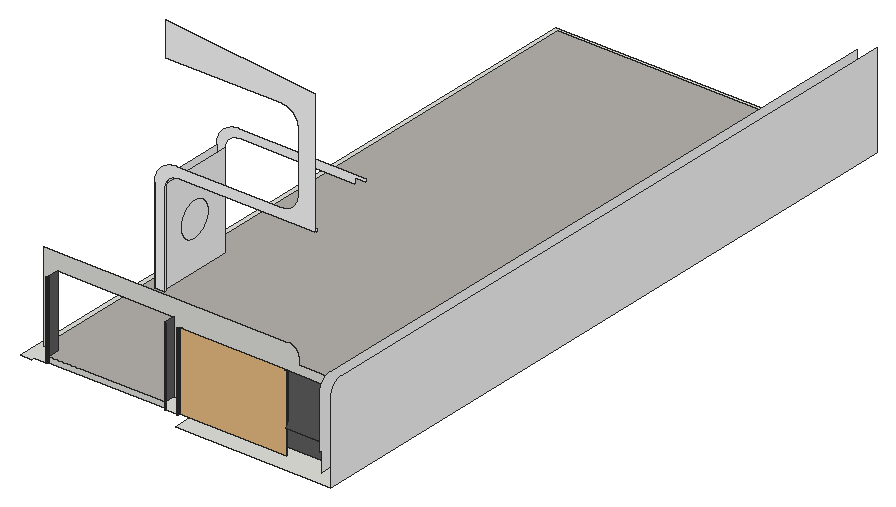
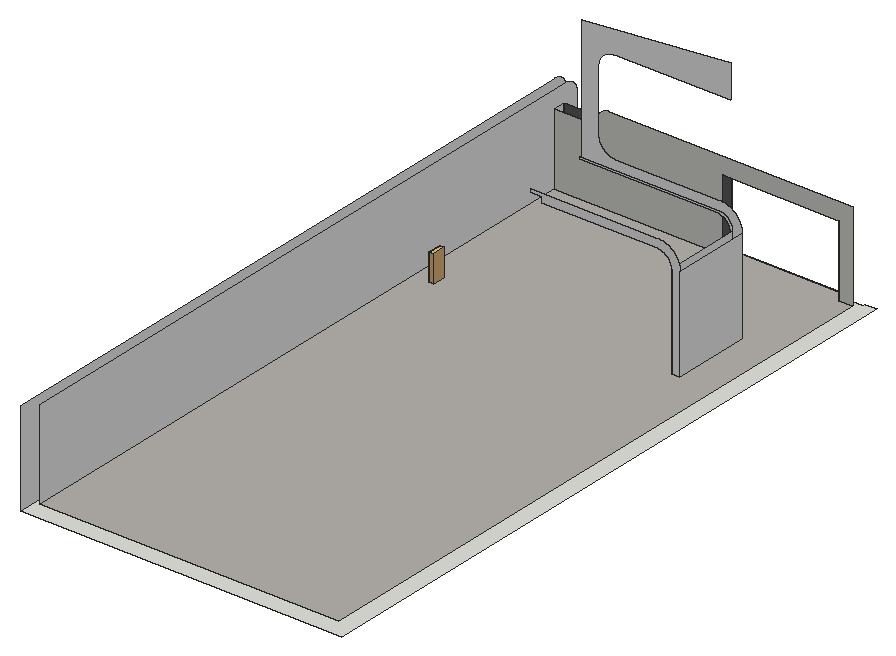
# SketchUp Ruby script. Lengths in inches.
U = 1.inch
M = Sketchup.active_model
def pt(a) = Geom::Point3d.new(a.map { |v| v * U })
def face(e, loops, mat)
  f = e.add_face(loops[0].map { |a| pt(a) })
  loops[1..].each { |l| e.add_face(l.map { |a| pt(a) }).erase! }
  f.material = f.back_material = mat if mat
  f
end
# faces: each face lists its corners as indices into pts; further lists are holes
def faces(e, pts, list, mat = nil) = list.each { |f| face(e, (f[0].is_a?(Array) ? f : [f]).map { |l| l.map { |i| pts[i] } }, mat) }
# xy, xz, yz: faces in a plane at the given z, y or x. An outline is a flat list of corners, or four numbers for a rectangle; further outlines are holes
def ring(l) = l.size == 4 ? [[l[0], l[1]], [l[2], l[1]], [l[2], l[3]], [l[0], l[3]]] : l.each_slice(2).to_a
def flat(e, list, mat, &to3) = list.each { |f| face(e, (f[0].is_a?(Array) ? f : [f]).map { |l| ring(l).map { |u, v| to3.(u, v) } }, mat) }
def xy(e, z, list, mat = nil) = flat(e, list, mat) { |x, y| [x, y, z] }
def xz(e, y, list, mat = nil) = flat(e, list, mat) { |x, z| [x, y, z] }
def yz(e, x, list, mat = nil) = flat(e, list, mat) { |y, z| [x, y, z] }
def lines(e, pts, list) = list.each { |a, b| e.add_line(pt(pts[a]), pt(pts[b])) }
# prism: a flat outline (further loops are holes) pulled along v
def prism(e, loops, v, mat = nil)
  f = face(e, loops, mat); d = Geom::Vector3d.new(v.map { |x| x * U })
  f.pushpull(f.normal.samedirection?(d) ? d.length : -d.length)
end
def box(e, o, s, mat = nil) = prism(e, [[o, [o[0] + s[0], o[1], o[2]], [o[0] + s[0], o[1] + s[1], o[2]], [o[0], o[1] + s[1], o[2]]]], [0, 0, s[2]], mat)
def at(x, y, z, deg = 0) = Geom::Transformation.translation(pt([x, y, z])) * Geom::Transformation.rotation(ORIGIN, Z_AXIS, deg.degrees)
def axes(o, x, y, z) = Geom::Transformation.new([*x, 0, *y, 0, *z, 0, *pt(o).to_a, 1])
def part(name) = M.definitions.add(name)
# library, detail: a bought-in or finely detailed component or shape, given as its bounding box
def library(name, o, s) = part(name).tap { |d| box(d.entities, o, s) }
def detail(e, o, s) = box(e.add_group.entities, o, s)
def put(e, d, t, mat = nil) = e.add_instance(d, t).tap { |i| i.material = mat if mat }
def group(e, t, mat = nil) = e.add_group.tap { |g| g.transformation = t; g.material = mat if mat }.entities
root = M.entities
M.materials.add("1421 AP 8232 ELEGANT GREY").color = [96, 96, 96]
M.materials.add("[Quartz Light Grey]").color = [251, 251, 252]
M.materials.add("[Tile Travertine 2 inch]").color = [181, 178, 172]
c1 = library("Group\#28",[0,-0.25,0],[115.92,0.25,83.97])
c2 = library("Group\#141",[-208.23,2037.18,75.37],[621.09,225.61,1251.82])
xy(root,-18,[[180,36,180,55,169,55,169,54.92,168.99,54.84,168.99,54.76,168.98,54.6875,168.96,54.61,168.94,54.53,168.92,54.46,168.9,54.38,168.875,54.31,168.85,54.23,168.82,54.16,168.74,54.02,168.71,53.96,168.66,53.89,168.62,53.82,168.47,53.64,168.41,53.59,168.36,53.53,168.18,53.38,168.11,53.34,168.04,53.29,167.98,53.26,167.84,53.18,167.77,53.15,167.69,53.125,167.62,53.1,167.54,53.08,167.47,53.06,167.39,53.04,167.3125,53.02,167.24,53.01,167.16,53.01,167.08,53,154.92,53,154.84,53.01,154.76,53.01,154.6875,53.02,154.61,53.04,154.53,53.06,154.46,53.08,154.38,53.1,154.31,53.125,154.23,53.15,154.16,53.18,154.02,53.26,153.96,53.29,153.89,53.34,153.82,53.38,153.64,53.53,153.59,53.59,153.53,53.64,153.38,53.82,153.34,53.89,153.29,53.96,153.26,54.02,153.18,54.16,153.15,54.23,153.125,54.31,153.1,54.38,153.08,54.46,153.06,54.53,153.04,54.61,153.02,54.6875,153.01,54.76,153.01,54.84,153,54.92,153,55,27,55,27,54.92,26.99,54.84,26.99,54.76,26.98,54.6875,26.96,54.61,26.94,54.53,26.92,54.46,26.9,54.38,26.875,54.31,26.85,54.23,26.82,54.16,26.74,54.02,26.71,53.96,26.66,53.89,26.62,53.82,26.47,53.64,26.41,53.59,26.36,53.53,26.18,53.38,26.11,53.34,26.04,53.29,25.98,53.26,25.84,53.18,25.77,53.15,25.69,53.125,25.62,53.1,25.54,53.08,25.47,53.06,25.39,53.04,25.3125,53.02,25.24,53.01,25.16,53.01,25.08,53,12,53,12,50,0,50,0,775,348,775,348,36]])
xy(root,-12,[[27,55,153,55,153,67,336,67,336,763,12,763,12,67,27,67]],"[Tile Travertine 2 inch]")
xy(root,0,[[36,187,36,271,45,271,45,189,47,189,47,187]],"[Quartz Light Grey]")
xy(root,9.97,[[284.92,53.5,336,55]])
xz(root,53,[[154.92,-18,155,66]],"1421 AP 8232 ELEGANT GREY")
xz(root,53.01,[[25.16,-18,25.24,66],[154.76,-18,154.84,66],[167.16,-18,167.24,65.97]],"1421 AP 8232 ELEGANT GREY")
xz(root,53.5,[[284.92,9.97,336,9.97,336,66,288,66,288,17.6875,287.99,17.53,287.98,17.37,287.97,17.22,287.95,16.9,287.93,16.75,287.92,16.59,287.9,16.43,287.875,16.28,287.85,16.12,287.83,15.97,287.8,15.8125,287.77,15.66,287.74,15.51,287.7,15.35,287.67,15.2,287.63,15.05,287.59,14.89,287.51,14.59,287.36,14.14,287.3125,13.99,287.26,13.85,287.2,13.7,287.15,13.55,287.09,13.41,287.03,13.26,286.96,13.12,286.9,12.98,286.83,12.83,286.55,12.27,286.47,12.14,286.39,12,286.3125,11.86,286.23,11.73,286.15,11.6,286.0625,11.46,285.98,11.33,285.8,11.07,285.71,10.95,285.62,10.82,285.52,10.69,285.42,10.57,285.33,10.45,285.23,10.33,285.02,10.09]],"1421 AP 8232 ELEGANT GREY")
xz(root,55,[[27,-18,153,-12]])
xz(root,55,[[169,-18,180,-18,180,-13.5,180.04,-12.91,180.15,-12.34,180.34,-11.78,180.6,-11.25,180.93,-10.76,181.32,-10.32,181.76,-9.93,182.25,-9.6,182.78,-9.34,183.34,-9.15,183.91,-9.04,184.5,-9,336,-9,336,9.97,284.92,9.97,284.8125,9.85,284.7,9.74,284.6,9.625,284.49,9.51,284.375,9.4,284.26,9.3,284.15,9.1875,284.03,9.08,283.91,8.98,283.67,8.77,283.55,8.67,283.43,8.58,283.31,8.48,283.18,8.38,283.05,8.29,282.93,8.2,282.67,8.02,282.54,7.9375,282.4,7.85,282.27,7.77,282.14,7.6875,282,7.61,281.86,7.53,281.73,7.45,281.17,7.17,281.02,7.1,280.88,7.04,280.74,6.97,280.59,6.91,280.45,6.85,280.3,6.8,280.15,6.74,280.01,6.6875,279.86,6.64,279.41,6.49,279.11,6.41,278.95,6.37,278.8,6.33,278.65,6.3,278.49,6.26,278.34,6.23,278.1875,6.2,278.03,6.17,277.88,6.15,277.72,6.125,277.57,6.1,277.41,6.08,277.25,6.07,277.1,6.05,276.78,6.03,276.63,6.02,276.47,6.01,276.3125,6,221.71,6,221.41,6.01,221.12,6.02,220.82,6.04,220.53,6.06,220.23,6.08,219.9375,6.11,219.65,6.14,219.35,6.18,219.0625,6.22,218.77,6.27,218.48,6.32,218.1875,6.37,217.9,6.43,217.32,6.55,217.04,6.62,216.75,6.69,216.47,6.77,216.18,6.85,215.9,6.9375,215.62,7.03,215.34,7.12,215.0625,7.22,214.78,7.32,214.51,7.42,214.23,7.53,213.96,7.64,213.15,8,212.89,8.13,212.36,8.39,212.1,8.53,211.84,8.68,211.59,8.82,211.33,8.97,210.83,9.28,210.58,9.44,210.34,9.6,210.09,9.77,209.61,10.11,209.38,10.29,209.14,10.47,208.91,10.65,208.68,10.84,208.24,11.22,207.58,11.82,207.37,12.03,207.16,12.23,206.96,12.45,206.75,12.66,206.55,12.875,206.36,13.1,206.16,13.32,205.97,13.54,205.78,13.77,205.42,14.23,205.24,14.47,204.9,14.95,204.73,15.1875,204.5625,15.43,204.4,15.68,204.25,15.93,204.09,16.18,203.94,16.4375,203.79,16.69,203.51,17.21,203.24,17.73,203.12,18,186,54,185.89,54.26,185.77,54.53,185.65,54.79,185.53,55.04,185.27,55.56,185.13,55.81,185,56.06,184.85,56.31,184.71,56.56,184.56,56.8,184.4,57.04,184.25,57.28,184.09,57.52,183.92,57.76,183.76,57.99,183.59,58.22,183.41,58.45,182.87,59.11,182.49,59.55,182.3,59.76,182.1,59.97,181.9,60.17,181.5,60.58,181.29,60.77,181.08,60.97,180.86,61.16,180.65,61.34,180.43,61.53,180.2,61.71,179.98,61.89,179.75,62.0625,179.52,62.23,179.29,62.4,179.05,62.5625,178.82,62.72,178.34,63.04,178.09,63.1875,177.84,63.33,177.6,63.48,177.35,63.61,177.09,63.75,176.84,63.88,176.58,64.01,176.32,64.13,176.0625,64.25,175.8,64.37,175.54,64.48,175.27,64.59,175.01,64.7,174.47,64.9,174.2,64.99,173.92,65.08,173.65,65.16,173.1,65.32,172.54,65.46,172.27,65.53,171.98,65.59,171.7,65.65,171.14,65.75,170.86,65.79,170.57,65.83,170.29,65.87,170,65.9,169.72,65.92,169.43,65.95,169.15,65.97,169,65.97]],"1421 AP 8232 ELEGANT GREY")
xz(root,67,[[12,-12,12,84,276.3125,84,276.47,83.99,276.63,83.98,276.78,83.97,277.1,83.95,277.25,83.93,277.41,83.92,277.57,83.9,277.72,83.875,277.88,83.85,278.03,83.83,278.1875,83.8,278.34,83.77,278.49,83.74,278.65,83.7,278.8,83.67,278.95,83.63,279.11,83.59,279.41,83.51,279.86,83.36,280.01,83.3125,280.15,83.26,280.3,83.2,280.45,83.15,280.59,83.09,280.74,83.03,280.88,82.96,281.02,82.9,281.17,82.83,281.73,82.55,281.86,82.47,282,82.39,282.14,82.3125,282.27,82.23,282.4,82.15,282.54,82.0625,282.67,81.98,282.93,81.8,283.05,81.71,283.18,81.62,283.31,81.52,283.43,81.42,283.55,81.33,283.67,81.23,283.91,81.02,284.03,80.92,284.15,80.8125,284.26,80.7,284.375,80.6,284.49,80.49,284.6,80.375,284.7,80.26,284.8125,80.15,284.92,80.03,285.02,79.91,285.23,79.67,285.33,79.55,285.42,79.43,285.52,79.31,285.62,79.18,285.71,79.05,285.8,78.93,285.98,78.67,286.0625,78.54,286.15,78.4,286.23,78.27,286.3125,78.14,286.39,78,286.47,77.86,286.55,77.73,286.83,77.17,286.9,77.02,286.96,76.88,287.03,76.74,287.09,76.59,287.15,76.45,287.2,76.3,287.26,76.15,287.3125,76.01,287.36,75.86,287.51,75.41,287.59,75.11,287.63,74.95,287.67,74.8,287.7,74.65,287.74,74.49,287.77,74.34,287.8,74.1875,287.83,74.03,287.85,73.88,287.875,73.72,287.9,73.57,287.92,73.41,287.93,73.25,287.95,73.1,287.97,72.78,287.98,72.63,287.99,72.47,288,72.3125,288,66,336,66,336,-12,153,-12,153,66,27,66,27,-12]])
xz(root,187,[[36,0,47,0,47,102.34,47.05,103.19,47.13,103.87,47.16,104.03,47.1875,104.2,47.22,104.37,47.25,104.54,47.28,104.7,47.32,104.87,47.36,105.03,47.4,105.2,47.44,105.36,47.49,105.53,47.54,105.69,47.58,105.86,47.64,106.02,47.69,106.18,47.75,106.34,47.8,106.5,47.86,106.66,47.93,106.82,47.99,106.97,48.06,107.13,48.125,107.29,48.19,107.44,48.27,107.6,48.34,107.75,48.74,108.5,48.83,108.65,48.92,108.79,49.01,108.9375,49.1,109.08,49.19,109.22,49.29,109.36,49.38,109.5,49.58,109.78,49.6875,109.91,49.79,110.05,49.9,110.18,50.01,110.3125,50.11,110.44,50.23,110.57,50.34,110.7,50.45,110.82,50.57,110.95,50.6875,111.07,50.81,111.19,50.93,111.3125,51.05,111.43,51.18,111.55,51.3,111.66,51.43,111.77,51.56,111.89,51.6875,111.99,51.82,112.1,51.95,112.21,52.09,112.3125,52.22,112.42,52.5,112.62,52.64,112.71,52.78,112.81,52.92,112.9,53.0625,112.99,53.21,113.08,53.35,113.17,53.5,113.26,54.25,113.66,54.4,113.73,54.56,113.81,54.71,113.875,54.87,113.94,55.03,114.01,55.18,114.07,55.34,114.14,55.5,114.2,55.66,114.25,55.82,114.31,55.98,114.36,56.14,114.42,56.31,114.46,56.47,114.51,56.64,114.56,56.8,114.6,56.97,114.64,57.13,114.68,57.3,114.72,57.46,114.75,57.63,114.78,57.8,114.8125,57.97,114.84,58.13,114.87,58.81,114.95,59.66,115,210,115,210,249,48,264,48,228,174.24,228,174.47,227.99,174.71,227.99,174.94,227.98,175.18,227.96,175.41,227.94,175.65,227.92,175.88,227.9,176.12,227.875,176.35,227.85,176.58,227.8125,176.82,227.78,177.28,227.7,177.51,227.65,177.74,227.61,177.97,227.56,178.2,227.5,178.43,227.45,178.66,227.39,178.89,227.32,179.11,227.26,179.34,227.19,179.5625,227.12,179.79,227.04,180.01,226.97,180.23,226.89,180.45,226.8,180.67,226.72,181.11,226.54,181.32,226.44,181.54,226.35,181.75,226.25,181.96,226.14,182.17,226.04,182.59,225.82,182.8,225.7,183,225.59,183.4,225.35,183.61,225.22,183.8,225.1,184,224.97,184.2,224.83,184.39,224.7,184.58,224.5625,184.77,224.42,184.96,224.28,185.14,224.14,185.33,223.99,185.51,223.84,185.69,223.6875,185.87,223.53,186.04,223.375,186.22,223.22,186.39,223.06,186.56,222.89,186.73,222.73,186.89,222.56,187.06,222.39,187.22,222.22,187.375,222.04,187.53,221.87,187.6875,221.69,187.84,221.51,187.99,221.33,188.14,221.14,188.28,220.96,188.42,220.77,188.5625,220.58,188.7,220.39,188.83,220.2,188.97,220,189.1,219.8,189.22,219.61,189.35,219.4,189.59,219,189.7,218.8,189.82,218.59,190.04,218.17,190.14,217.96,190.25,217.75,190.35,217.54,190.44,217.32,190.54,217.11,190.72,216.67,190.8,216.45,190.89,216.23,190.97,216.01,191.04,215.79,191.12,215.5625,191.19,215.34,191.26,215.11,191.32,214.89,191.39,214.66,191.45,214.43,191.5,214.2,191.56,213.97,191.61,213.74,191.65,213.51,191.7,213.28,191.78,212.82,191.8125,212.58,191.85,212.35,191.875,212.12,191.9,211.88,191.92,211.65,191.94,211.41,191.96,211.18,191.98,210.94,191.99,210.71,191.99,210.47,192,210.24,192,143.76,191.99,143.53,191.99,143.29,191.98,143.06,191.96,142.82,191.94,142.59,191.92,142.35,191.9,142.12,191.875,141.88,191.85,141.65,191.8125,141.42,191.78,141.18,191.7,140.72,191.65,140.49,191.61,140.26,191.56,140.03,191.5,139.8,191.45,139.57,191.39,139.34,191.32,139.11,191.26,138.89,191.19,138.66,191.12,138.4375,191.04,138.21,190.97,137.99,190.89,137.77,190.8,137.55,190.72,137.33,190.54,136.89,190.44,136.68,190.35,136.46,190.25,136.25,190.14,136.04,190.04,135.83,189.82,135.41,189.7,135.2,189.59,135,189.35,134.6,189.22,134.39,189.1,134.2,188.97,134,188.83,133.8,188.7,133.61,188.5625,133.42,188.42,133.23,188.28,133.04,188.14,132.86,187.99,132.67,187.84,132.49,187.6875,132.31,187.53,132.13,187.375,131.96,187.22,131.78,187.06,131.61,186.89,131.44,186.73,131.27,186.56,131.11,186.39,130.94,186.22,130.78,186.04,130.625,185.87,130.47,185.69,130.3125,185.51,130.16,185.33,130.01,185.14,129.86,184.96,129.72,184.77,129.58,184.58,129.4375,184.39,129.3,184.2,129.17,184,129.03,183.94,128.99,183.8,128.9,183.61,128.78,183.4,128.65,183,128.41,182.8,128.3,182.59,128.18,182.17,127.96,181.96,127.86,181.75,127.75,181.54,127.65,181.32,127.56,181.11,127.46,180.67,127.28,180.45,127.2,180.23,127.11,180.01,127.03,179.79,126.96,179.5625,126.88,179.34,126.81,179.11,126.74,178.89,126.68,178.66,126.61,178.43,126.55,178.2,126.5,177.97,126.44,177.74,126.39,177.51,126.35,177.28,126.3,176.82,126.22,176.58,126.1875,176.35,126.15,176.12,126.125,175.88,126.1,175.65,126.08,175.41,126.06,175.18,126.04,174.94,126.02,174.71,126.01,174.47,126.01,174.24,126,59.6875,126,59.37,125.99,59.06,125.98,58.74,125.97,58.12,125.93,57.8,125.9,57.49,125.87,56.56,125.75,56.25,125.7,55.625,125.6,55.32,125.54,55.01,125.48,54.7,125.41,54.4,125.34,54.09,125.26,53.49,125.1,53.18,125.01,52.58,124.83,52.29,124.73,51.69,124.52,51.4,124.41,50.24,123.93,49.95,123.8,49.39,123.52,49.1,123.38,48.83,123.24,48.27,122.94,48,122.78,47.73,122.625,47.46,122.46,47.19,122.3,46.67,121.96,45.89,121.42,45.14,120.85,44.9,120.65,44.65,120.45,44.41,120.25,44.18,120.04,43.94,119.84,43.48,119.41,43.25,119.19,42.81,118.75,42.59,118.52,42.16,118.06,41.96,117.82,41.75,117.59,41.55,117.35,41.35,117.1,41.15,116.86,40.58,116.11,40.04,115.33,39.7,114.81,39.54,114.54,39.375,114.27,39.22,114,39.06,113.73,38.76,113.17,38.62,112.9,38.48,112.61,38.2,112.05,38.07,111.76,37.59,110.6,37.48,110.31,37.27,109.71,37.17,109.42,36.99,108.82,36.9,108.51,36.74,107.91,36.66,107.6,36.59,107.3,36.52,106.99,36.46,106.68,36.4,106.375,36.3,105.75,36.25,105.44,36.13,104.51,36.1,104.2,36.07,103.88,36.03,103.26,36.02,102.94,36.01,102.63,36,102.3125]],"[Quartz Light Grey]")
xz(root,189,[[45,0,45,102.2,45.01,102.39,45.01,102.59,45.02,102.79,45.03,102.98,45.05,103.18,45.0625,103.37,45.08,103.57,45.1,103.76,45.13,103.96,45.16,104.15,45.18,104.35,45.22,104.54,45.25,104.73,45.29,104.93,45.41,105.5,45.51,105.88,45.5625,106.07,45.62,106.26,45.67,106.45,45.73,106.64,45.8,106.82,45.86,107.01,45.93,107.19,46.07,107.56,46.14,107.74,46.46,108.46,46.55,108.63,46.63,108.81,46.73,108.98,46.82,109.16,46.91,109.33,47.21,109.84,47.3125,110,47.42,110.17,47.53,110.33,47.64,110.5,47.86,110.82,47.98,110.97,48.22,111.29,48.34,111.44,48.47,111.59,48.59,111.74,48.85,112.04,48.99,112.18,49.12,112.33,49.26,112.47,49.39,112.61,49.53,112.74,49.67,112.88,49.82,113.01,49.96,113.15,50.26,113.41,50.41,113.53,50.56,113.66,50.71,113.78,51.03,114.02,51.18,114.14,51.5,114.36,51.67,114.47,51.83,114.58,52,114.6875,52.16,114.79,52.67,115.09,52.84,115.18,53.02,115.27,53.19,115.37,53.37,115.45,53.54,115.54,54.26,115.86,54.44,115.93,54.81,116.07,54.99,116.14,55.18,116.2,55.36,116.27,55.55,116.33,55.74,116.38,55.93,116.4375,56.12,116.49,56.5,116.59,57.07,116.71,57.27,116.75,57.46,116.78,57.65,116.82,57.85,116.84,58.04,116.87,58.24,116.9,58.43,116.92,58.63,116.9375,58.82,116.95,59.02,116.97,59.21,116.98,59.41,116.99,59.61,116.99,59.8,117,210,117,210,115,59.66,115,58.81,114.95,58.13,114.87,57.97,114.84,57.8,114.8125,57.63,114.78,57.46,114.75,57.3,114.72,57.13,114.68,56.97,114.64,56.8,114.6,56.64,114.56,56.47,114.51,56.31,114.46,56.14,114.42,55.98,114.36,55.82,114.31,55.66,114.25,55.5,114.2,55.34,114.14,55.18,114.07,55.03,114.01,54.87,113.94,54.71,113.875,54.56,113.81,54.4,113.73,54.25,113.66,53.5,113.26,53.35,113.17,53.21,113.08,53.0625,112.99,52.92,112.9,52.78,112.81,52.64,112.71,52.5,112.62,52.22,112.42,52.09,112.3125,51.95,112.21,51.82,112.1,51.6875,111.99,51.56,111.89,51.43,111.77,51.3,111.66,51.18,111.55,51.05,111.43,50.93,111.3125,50.81,111.19,50.6875,111.07,50.57,110.95,50.45,110.82,50.34,110.7,50.23,110.57,50.11,110.44,50.01,110.3125,49.9,110.18,49.79,110.05,49.6875,109.91,49.58,109.78,49.38,109.5,49.29,109.36,49.19,109.22,49.1,109.08,49.01,108.9375,48.92,108.79,48.83,108.65,48.74,108.5,48.34,107.75,48.27,107.6,48.19,107.44,48.125,107.29,48.06,107.13,47.99,106.97,47.93,106.82,47.86,106.66,47.8,106.5,47.75,106.34,47.69,106.18,47.64,106.02,47.58,105.86,47.54,105.69,47.49,105.53,47.44,105.36,47.4,105.2,47.36,105.03,47.32,104.87,47.28,104.7,47.25,104.54,47.22,104.37,47.1875,104.2,47.16,104.03,47.13,103.87,47.05,103.19,47,102.34,47,0]],"[Quartz Light Grey]")
xz(root,271,[[36,0,36,102.3125,36.01,102.63,36.02,102.94,36.03,103.26,36.07,103.88,36.1,104.2,36.13,104.51,36.25,105.44,36.3,105.75,36.4,106.375,36.46,106.68,36.52,106.99,36.59,107.3,36.66,107.6,36.74,107.91,36.9,108.51,36.99,108.82,37.17,109.42,37.27,109.71,37.48,110.31,37.59,110.6,38.07,111.76,38.2,112.05,38.48,112.61,38.62,112.9,38.76,113.17,39.06,113.73,39.22,114,39.375,114.27,39.54,114.54,39.7,114.81,40.04,115.33,40.58,116.11,41.15,116.86,41.35,117.1,41.55,117.35,41.75,117.59,41.96,117.82,42.16,118.06,42.59,118.52,42.81,118.75,43.25,119.19,43.48,119.41,43.94,119.84,44.18,120.04,44.41,120.25,44.65,120.45,44.9,120.65,45.14,120.85,45.89,121.42,46.67,121.96,47.19,122.3,47.46,122.46,47.73,122.625,48,122.78,48.27,122.94,48.83,123.24,49.1,123.38,49.39,123.52,49.95,123.8,50.24,123.93,51.4,124.41,51.69,124.52,52.29,124.73,52.58,124.83,53.18,125.01,53.49,125.1,54.09,125.26,54.4,125.34,54.7,125.41,55.01,125.48,55.32,125.54,55.625,125.6,56.25,125.7,56.56,125.75,57.49,125.87,57.8,125.9,58.12,125.93,58.74,125.97,59.06,125.98,59.37,125.99,59.6875,126,198,126,198,123,186,123,186,117,59.8,117,59.61,116.99,59.41,116.99,59.21,116.98,59.02,116.97,58.82,116.95,58.63,116.9375,58.43,116.92,58.24,116.9,58.04,116.87,57.85,116.84,57.65,116.82,57.46,116.78,57.27,116.75,57.07,116.71,56.5,116.59,56.12,116.49,55.93,116.4375,55.74,116.38,55.55,116.33,55.36,116.27,55.18,116.2,54.99,116.14,54.81,116.07,54.44,115.93,54.26,115.86,53.54,115.54,53.37,115.45,53.19,115.37,53.02,115.27,52.84,115.18,52.67,115.09,52.16,114.79,52,114.6875,51.83,114.58,51.67,114.47,51.5,114.36,51.18,114.14,51.03,114.02,50.71,113.78,50.56,113.66,50.41,113.53,50.26,113.41,49.96,113.15,49.82,113.01,49.67,112.88,49.53,112.74,49.39,112.61,49.26,112.47,49.12,112.33,48.99,112.18,48.85,112.04,48.59,111.74,48.47,111.59,48.34,111.44,48.22,111.29,47.98,110.97,47.86,110.82,47.64,110.5,47.53,110.33,47.42,110.17,47.3125,110,47.21,109.84,46.91,109.33,46.82,109.16,46.73,108.98,46.63,108.81,46.55,108.63,46.46,108.46,46.14,107.74,46.07,107.56,45.93,107.19,45.86,107.01,45.8,106.82,45.73,106.64,45.67,106.45,45.62,106.26,45.5625,106.07,45.51,105.88,45.41,105.5,45.29,104.93,45.25,104.73,45.22,104.54,45.18,104.35,45.16,104.15,45.13,103.96,45.1,103.76,45.08,103.57,45.0625,103.37,45.05,103.18,45.03,102.98,45.02,102.79,45.01,102.59,45.01,102.39,45,102.2,45,0]],"[Quartz Light Grey]")
yz(root,26.99,[[54.76,-18,54.84,66]],"1421 AP 8232 ELEGANT GREY")
yz(root,27,[[54.92,-18,55,66],[55,-12,67,66]],"1421 AP 8232 ELEGANT GREY")
yz(root,36,[[187,0,271,102]],"[Quartz Light Grey]")
yz(root,45,[[[189,0,271,102],[229.9375,32,229.44,32.01,228.94,32.03,228.45,32.0625,227.95,32.11,227.46,32.17,226.97,32.24,226.48,32.33,225.99,32.43,225.5,32.54,225.02,32.66,224.54,32.8,224.07,32.95,223.6,33.11,223.13,33.28,222.67,33.47,222.22,33.67,221.76,33.88,221.32,34.1,220.88,34.33,220.02,34.83,219.6,35.1,219.1875,35.375,218.78,35.67,218.38,35.96,217.99,36.27,217.61,36.59,217.24,36.92,216.875,37.26,216.52,37.61,215.84,38.33,215.51,38.71,215.2,39.09,214.89,39.48,214.59,39.88,214.03,40.7,213.51,41.55,213.27,41.99,213.04,42.43,212.82,42.875,212.62,43.33,212.42,43.79,212.24,44.25,212.07,44.72,211.91,45.1875,211.76,45.66,211.63,46.14,211.51,46.625,211.4,47.11,211.22,48.09,211.15,48.58,211.1,49.08,211.05,49.57,211.02,50.07,211,50.56,211,51.0625,211.01,51.56,211.03,52.06,211.0625,52.55,211.11,53.05,211.17,53.54,211.24,54.03,211.33,54.52,211.43,55.01,211.54,55.5,211.66,55.98,211.8,56.46,211.95,56.93,212.11,57.4,212.28,57.87,212.47,58.33,212.67,58.78,212.88,59.24,213.1,59.68,213.33,60.12,213.83,60.98,214.1,61.4,214.375,61.8125,214.67,62.22,214.96,62.62,215.27,63.01,215.59,63.39,215.92,63.76,216.26,64.125,216.61,64.48,217.33,65.16,217.71,65.49,218.09,65.8,218.48,66.11,218.88,66.41,219.7,66.97,220.55,67.49,220.99,67.73,221.43,67.96,221.875,68.18,222.33,68.38,222.79,68.58,223.25,68.76,223.72,68.93,224.1875,69.09,224.66,69.24,225.14,69.37,225.625,69.49,226.11,69.6,227.09,69.78,227.58,69.85,228.08,69.9,228.57,69.95,229.07,69.98,229.56,70,230.0625,70,230.56,69.99,231.06,69.97,231.55,69.9375,232.05,69.89,232.54,69.83,233.03,69.76,233.52,69.67,234.01,69.57,234.5,69.46,234.98,69.34,235.46,69.2,235.93,69.05,236.4,68.89,236.87,68.72,237.33,68.53,237.78,68.33,238.24,68.12,238.68,67.9,239.12,67.67,239.98,67.17,240.4,66.9,240.8125,66.625,241.22,66.33,241.62,66.04,242.01,65.73,242.39,65.41,242.76,65.08,243.125,64.74,243.48,64.39,244.16,63.67,244.49,63.29,244.8,62.91,245.11,62.52,245.41,62.12,245.97,61.3,246.49,60.45,246.73,60.01,246.96,59.57,247.18,59.125,247.38,58.67,247.58,58.21,247.76,57.75,247.93,57.28,248.09,56.8125,248.24,56.34,248.37,55.86,248.49,55.375,248.6,54.89,248.78,53.91,248.85,53.42,248.9,52.92,248.95,52.43,248.98,51.93,249,51.44,249,50.9375,248.99,50.44,248.97,49.94,248.9375,49.45,248.89,48.95,248.83,48.46,248.76,47.97,248.67,47.48,248.57,46.99,248.46,46.5,248.34,46.02,248.2,45.54,248.05,45.07,247.89,44.6,247.72,44.13,247.53,43.67,247.33,43.22,247.12,42.76,246.9,42.32,246.67,41.88,246.17,41.02,245.9,40.6,245.625,40.1875,245.33,39.78,245.04,39.38,244.73,38.99,244.41,38.61,244.08,38.24,243.74,37.875,243.39,37.52,242.67,36.84,242.29,36.51,241.91,36.2,241.52,35.89,241.12,35.59,240.3,35.03,239.45,34.51,239.01,34.27,238.57,34.04,238.125,33.82,237.67,33.62,237.21,33.42,236.75,33.24,236.28,33.07,235.8125,32.91,235.34,32.76,234.86,32.63,234.375,32.51,233.89,32.4,232.91,32.22,232.42,32.15,231.92,32.1,231.43,32.05,230.93,32.02,230.44,32]]],"[Quartz Light Grey]")
yz(root,47,[[187,0,189,102]],"[Quartz Light Grey]")
yz(root,153,[[54.92,-18,55,66],[55,-12,67,66]],"1421 AP 8232 ELEGANT GREY")
yz(root,153.01,[[54.76,-18,54.84,66]],"1421 AP 8232 ELEGANT GREY")
yz(root,168.99,[[54.76,-18,54.84,65.97]],"1421 AP 8232 ELEGANT GREY")
yz(root,169,[[54.92,-18,55,65.97]],"1421 AP 8232 ELEGANT GREY")
yz(root,336,[[67,-12,67,66,53.5,66,53.5,9.97,55,9.97,55,-9,39,-9,39,12,36,12,36,69.2,36.01,69.39,36.01,69.59,36.02,69.79,36.03,69.98,36.05,70.18,36.0625,70.37,36.08,70.57,36.1,70.76,36.13,70.96,36.16,71.15,36.18,71.35,36.22,71.54,36.25,71.73,36.29,71.93,36.41,72.5,36.51,72.88,36.5625,73.07,36.62,73.26,36.67,73.45,36.73,73.64,36.8,73.82,36.86,74.01,36.93,74.19,37.07,74.56,37.14,74.74,37.46,75.46,37.55,75.63,37.63,75.81,37.73,75.98,37.82,76.16,37.91,76.33,38.21,76.84,38.3125,77,38.42,77.17,38.53,77.33,38.64,77.5,38.86,77.82,38.98,77.97,39.22,78.29,39.34,78.44,39.47,78.59,39.59,78.74,39.85,79.04,39.99,79.18,40.12,79.33,40.26,79.47,40.39,79.61,40.53,79.74,40.67,79.88,40.82,80.01,40.96,80.15,41.26,80.41,41.41,80.53,41.56,80.66,41.71,80.78,42.03,81.02,42.18,81.14,42.5,81.36,42.67,81.47,42.83,81.58,43,81.6875,43.16,81.79,43.67,82.09,43.84,82.18,44.02,82.27,44.19,82.37,44.37,82.45,44.54,82.54,45.26,82.86,45.44,82.93,45.81,83.07,45.99,83.14,46.18,83.2,46.36,83.27,46.55,83.33,46.74,83.38,46.93,83.4375,47.12,83.49,47.5,83.59,48.07,83.71,48.27,83.75,48.46,83.78,48.65,83.82,48.85,83.84,49.04,83.87,49.24,83.9,49.43,83.92,49.63,83.9375,49.82,83.95,50.02,83.97,50.21,83.98,50.41,83.99,50.61,83.99,50.8,84,763,84,763,-12]],"[Quartz Light Grey]")
yz(root,348,[[36,-18,775,-18,775,84,50.8,84,50.61,83.99,50.41,83.99,50.21,83.98,50.02,83.97,49.82,83.95,49.63,83.9375,49.43,83.92,49.24,83.9,49.04,83.87,48.85,83.84,48.65,83.82,48.46,83.78,48.27,83.75,48.07,83.71,47.5,83.59,47.12,83.49,46.93,83.4375,46.74,83.38,46.55,83.33,46.36,83.27,46.18,83.2,45.99,83.14,45.81,83.07,45.44,82.93,45.26,82.86,44.54,82.54,44.37,82.45,44.19,82.37,44.02,82.27,43.84,82.18,43.67,82.09,43.16,81.79,43,81.6875,42.83,81.58,42.67,81.47,42.5,81.36,42.18,81.14,42.03,81.02,41.71,80.78,41.56,80.66,41.41,80.53,41.26,80.41,40.96,80.15,40.82,80.01,40.67,79.88,40.53,79.74,40.39,79.61,40.26,79.47,40.12,79.33,39.99,79.18,39.85,79.04,39.59,78.74,39.47,78.59,39.34,78.44,39.22,78.29,38.98,77.97,38.86,77.82,38.64,77.5,38.53,77.33,38.42,77.17,38.3125,77,38.21,76.84,37.91,76.33,37.82,76.16,37.73,75.98,37.63,75.81,37.55,75.63,37.46,75.46,37.14,74.74,37.07,74.56,36.93,74.19,36.86,74.01,36.8,73.82,36.73,73.64,36.67,73.45,36.62,73.26,36.5625,73.07,36.51,72.88,36.41,72.5,36.29,71.93,36.25,71.73,36.22,71.54,36.18,71.35,36.16,71.15,36.13,70.96,36.1,70.76,36.08,70.57,36.0625,70.37,36.05,70.18,36.03,70,36.03,69.98,36.02,69.79,36.01,69.59,36.01,69.39,36,69.2]],"[Quartz Light Grey]")
p = [[25.08,53,-18],[25.16,53.01,-18],[25.16,53.01,66],[25.08,53,66],[25.24,53.01,-18],[25.3125,53.02,-18],
  [25.3125,53.02,66],[25.24,53.01,66],[25.39,53.04,-18],[25.39,53.04,66],[25.47,53.06,-18],[25.47,53.06,66],
  [154.53,53.06,-18],[154.61,53.04,-18],[154.61,53.04,66],[154.53,53.06,66],[154.6875,53.02,-18],[154.6875,53.02,66],
  [154.76,53.01,-18],[154.76,53.01,66],[154.84,53.01,-18],[154.92,53,-18],[154.92,53,66],[154.84,53.01,66],
  [167.08,53,-18],[167.16,53.01,-18],[167.16,53.01,65.97],[167.08,53,65.97],[167.24,53.01,-18],[167.3125,53.02,-18],
  [167.3125,53.02,65.97],[167.24,53.01,65.97],[167.39,53.04,-18],[167.39,53.04,65.97],[167.47,53.06,-18],[167.47,53.06,65.97],
  [25.54,53.08,-18],[25.54,53.08,66],[25.62,53.1,-18],[25.62,53.1,66],[25.69,53.125,-18],[25.69,53.125,66],
  [25.77,53.15,-18],[25.77,53.15,66],[154.23,53.15,-18],[154.31,53.125,-18],[154.31,53.125,66],[154.23,53.15,66],
  [154.38,53.1,-18],[154.38,53.1,66],[154.46,53.08,-18],[154.46,53.08,66],[167.54,53.08,-18],[167.54,53.08,65.97],
  [167.62,53.1,-18],[167.62,53.1,65.97],[167.69,53.125,-18],[167.69,53.125,65.97],[167.77,53.15,-18],[167.77,53.15,65.97],
  [25.84,53.18,-18],[25.84,53.18,66],[25.91,53.22,-18],[25.91,53.22,66],[25.98,53.26,-18],[25.98,53.26,66],
  [154.02,53.26,-18],[154.09,53.22,-18],[154.09,53.22,66],[154.02,53.26,66],[154.16,53.18,-18],[154.16,53.18,66],
  [167.84,53.18,-18],[167.84,53.18,65.97],[167.91,53.22,-18],[167.91,53.22,65.97],[167.98,53.26,-18],[167.98,53.26,65.97],
  [26.04,53.29,-18],[26.04,53.29,66],[26.11,53.34,-18],[26.11,53.34,66],[26.18,53.38,-18],[26.18,53.38,66],
  [153.82,53.38,-18],[153.89,53.34,-18],[153.89,53.34,66],[153.82,53.38,66],[153.96,53.29,-18],[153.96,53.29,66],
  [168.04,53.29,-18],[168.04,53.29,65.97],[168.11,53.34,-18],[168.11,53.34,65.97],[168.18,53.38,-18],[168.18,53.38,65.97],
  [26.24,53.43,-18],[26.24,53.43,66],[26.3,53.48,-18],[26.3,53.48,66],[153.7,53.48,-18],[153.76,53.43,-18],
  [153.76,53.43,66],[153.7,53.48,66],[168.24,53.43,-18],[168.24,53.43,65.97],[168.3,53.48,-18],[168.3,53.48,65.97],
  [26.36,53.53,-18],[26.36,53.53,66],[26.41,53.59,-18],[26.41,53.59,66],[153.64,53.53,-18],[153.64,53.53,66],
  [153.59,53.59,-18],[153.59,53.59,66],[168.36,53.53,-18],[168.36,53.53,65.97],[168.41,53.59,-18],[168.41,53.59,65.97],
  [26.47,53.64,-18],[26.47,53.64,66],[26.52,53.7,-18],[26.52,53.7,66],[153.53,53.64,-18],[153.53,53.64,66],
  [153.48,53.7,-18],[153.48,53.7,66],[168.47,53.64,-18],[168.47,53.64,65.97],[168.52,53.7,-18],[168.52,53.7,65.97],
  [26.57,53.76,-18],[26.57,53.76,66],[153.43,53.76,-18],[153.43,53.76,66],[168.57,53.76,-18],[168.57,53.76,65.97],
  [26.62,53.82,-18],[26.62,53.82,66],[26.66,53.89,-18],[26.66,53.89,66],[153.34,53.89,-18],[153.38,53.82,-18],
  [153.38,53.82,66],[153.34,53.89,66],[168.62,53.82,-18],[168.62,53.82,65.97],[168.66,53.89,-18],[168.66,53.89,65.97],
  [26.71,53.96,-18],[26.71,53.96,66],[153.29,53.96,-18],[153.29,53.96,66],[168.71,53.96,-18],[168.71,53.96,65.97],
  [26.74,54.02,-18],[26.74,54.02,66],[26.78,54.09,-18],[26.78,54.09,66],[153.22,54.09,-18],[153.26,54.02,-18],
  [153.26,54.02,66],[153.22,54.09,66],[168.74,54.02,-18],[168.74,54.02,65.97],[168.78,54.09,-18],[168.78,54.09,65.97],
  [26.82,54.16,-18],[26.82,54.16,66],[153.18,54.16,-18],[153.18,54.16,66],[168.82,54.16,-18],[168.82,54.16,65.97],
  [26.85,54.23,-18],[26.85,54.23,66],[26.875,54.31,-18],[26.875,54.31,66],[153.125,54.31,-18],[153.15,54.23,-18],
  [153.15,54.23,66],[153.125,54.31,66],[168.85,54.23,-18],[168.85,54.23,65.97],[168.875,54.31,-18],[168.875,54.31,65.97],
  [26.9,54.38,-18],[26.9,54.38,66],[153.1,54.38,-18],[153.1,54.38,66],[168.9,54.38,-18],[168.9,54.38,65.97],
  [26.92,54.46,-18],[26.92,54.46,66],[153.08,54.46,-18],[153.08,54.46,66],[168.92,54.46,-18],[168.92,54.46,65.97],
  [26.94,54.53,-18],[26.94,54.53,66],[26.96,54.61,-18],[26.96,54.61,66],[153.04,54.61,-18],[153.06,54.53,-18],
  [153.06,54.53,66],[153.04,54.61,66],[168.94,54.53,-18],[168.94,54.53,65.97],[168.96,54.61,-18],[168.96,54.61,65.97],
  [26.98,54.6875,-18],[26.98,54.6875,66],[153.02,54.6875,-18],[153.02,54.6875,66],[168.98,54.6875,-18],[168.98,54.6875,65.97],
  [26.99,54.76,-18],[26.99,54.76,66],[153.01,54.76,-18],[153.01,54.76,66],[168.99,54.76,-18],[168.99,54.76,65.97],
  [26.99,54.84,-18],[27,54.92,-18],[27,54.92,66],[26.99,54.84,66],[153,54.92,-18],[153.01,54.84,-18],
  [153.01,54.84,66],[153,54.92,66],[168.99,54.84,-18],[169,54.92,-18],[169,54.92,65.97],[168.99,54.84,65.97]]
faces(root,p,[[0,1,2,3],[4,5,6,7],[5,8,9,6],[8,10,11,9],[12,13,14,15],[13,16,17,14],[16,18,19,17],[20,21,22,23],
  [24,25,26,27],[28,29,30,31],[29,32,33,30],[32,34,35,33],[10,36,37,11],[36,38,39,37],[38,40,41,39],[40,42,43,41],
  [44,45,46,47],[45,48,49,46],[48,50,51,49],[50,12,15,51],[34,52,53,35],[52,54,55,53],[54,56,57,55],[56,58,59,57],
  [42,60,61,43],[60,62,63,61],[62,64,65,63],[66,67,68,69],[67,70,71,68],[70,44,47,71],[58,72,73,59],[72,74,75,73],
  [74,76,77,75],[64,78,79,65],[78,80,81,79],[80,82,83,81],[84,85,86,87],[85,88,89,86],[88,66,69,89],[76,90,91,77],
  [90,92,93,91],[92,94,95,93],[82,96,97,83],[96,98,99,97],[100,101,102,103],[101,84,87,102],[94,104,105,95],[104,106,107,105],
  [98,108,109,99],[108,110,111,109],[112,100,103,113],[114,112,113,115],[106,116,117,107],[116,118,119,117],[110,120,121,111],[120,122,123,121],
  [124,114,115,125],[126,124,125,127],[118,128,129,119],[128,130,131,129],[122,132,133,123],[134,126,127,135],[130,136,137,131],[132,138,139,133],
  [138,140,141,139],[142,143,144,145],[143,134,135,144],[136,146,147,137],[146,148,149,147],[140,150,151,141],[152,142,145,153],[148,154,155,149],
  [150,156,157,151],[156,158,159,157],[160,161,162,163],[161,152,153,162],[154,164,165,155],[164,166,167,165],[158,168,169,159],[170,160,163,171],
  [166,172,173,167],[168,174,175,169],[174,176,177,175],[178,179,180,181],[179,170,171,180],[172,182,183,173],[182,184,185,183],[176,186,187,177],
  [188,178,181,189],[184,190,191,185],[186,192,193,187],[194,188,189,195],[190,196,197,191],[192,198,199,193],[198,200,201,199],[202,203,204,205],
  [203,194,195,204],[196,206,207,197],[206,208,209,207],[200,210,211,201],[212,202,205,213],[208,214,215,209],[210,216,217,211],[218,212,213,219],
  [214,220,221,215],[222,223,224,225],[226,227,228,229],[230,231,232,233]],"1421 AP 8232 ELEGANT GREY")
put(root,c1,at(169,55,-18),"1421 AP 8232 ELEGANT GREY")
put(root,c2,axes([253.68,273.14,0.11],[0,-0.02318,0],[0.02157,0,0],[0,0,0.02333]))
